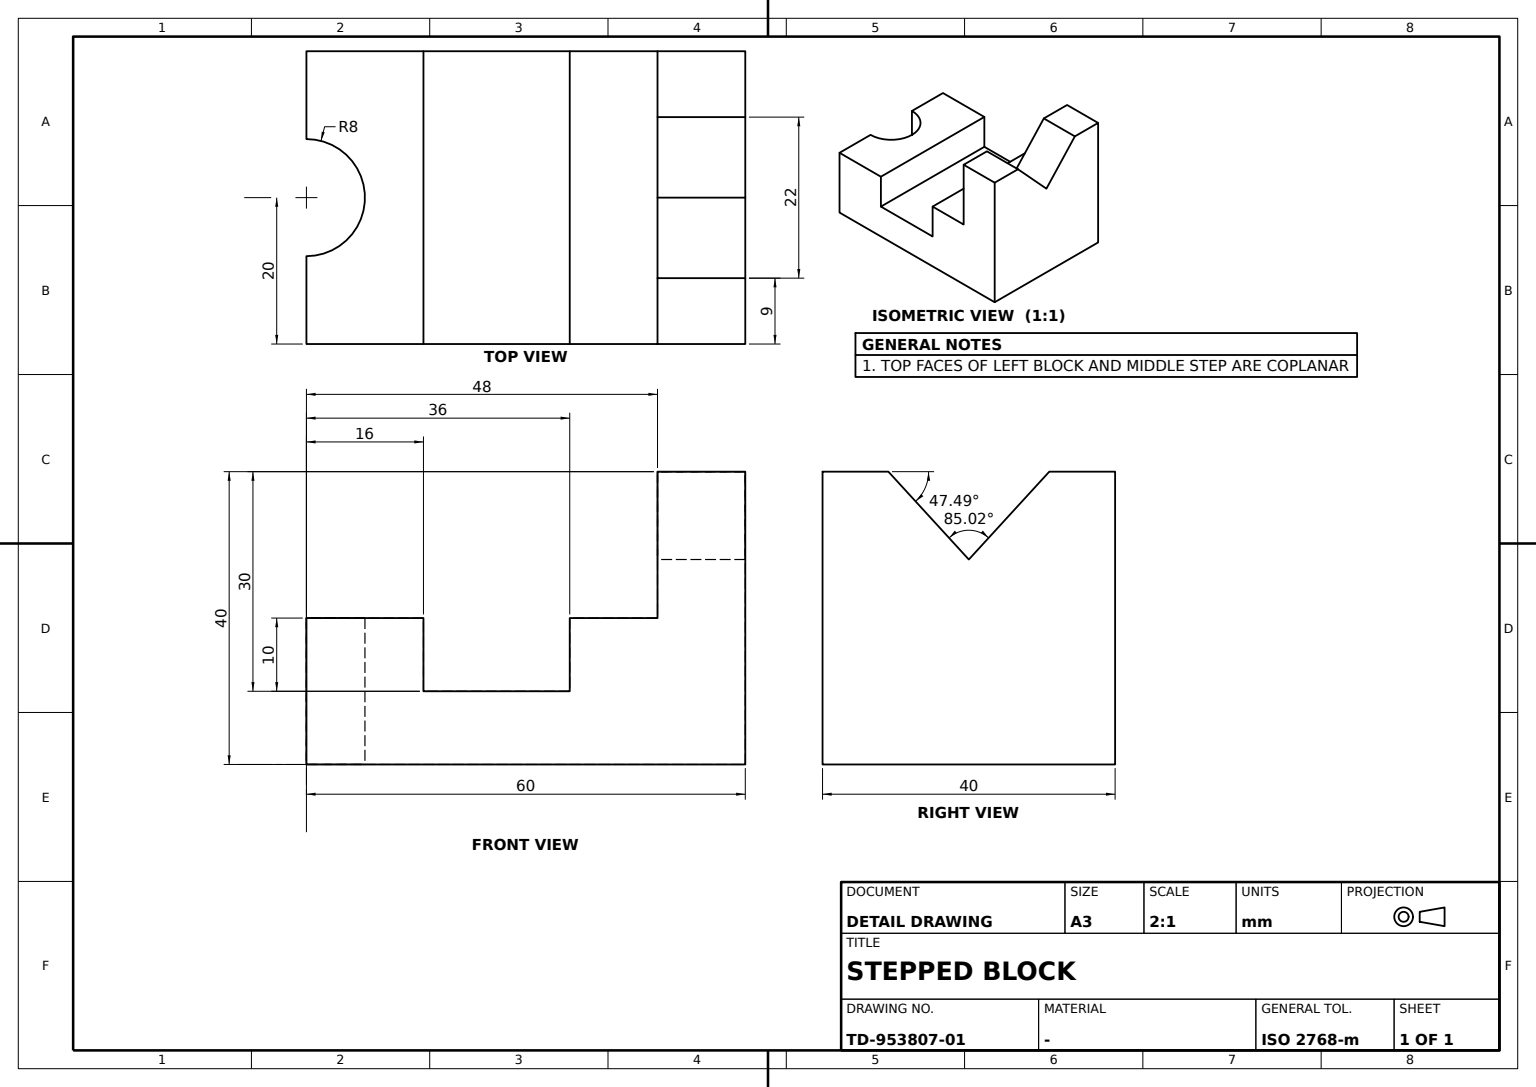
ISO-10303-21;
HEADER;
FILE_DESCRIPTION((''),'2;1');
FILE_NAME('','',(''),(''),'','','');
FILE_SCHEMA(('AUTOMOTIVE_DESIGN'));
ENDSEC;
DATA;
#1=APPLICATION_CONTEXT('');
#2=PRODUCT_CONTEXT('',#1,'mechanical');
#3=PRODUCT('','','',(#2));
#4=PRODUCT_DEFINITION_FORMATION('','',#3);
#5=PRODUCT_DEFINITION_CONTEXT('',#1,'design');
#6=PRODUCT_DEFINITION('','',#4,#5);
#7=PRODUCT_DEFINITION_SHAPE('','',#6);
#8=(LENGTH_UNIT()NAMED_UNIT(*)SI_UNIT(.MILLI.,.METRE.));
#9=(NAMED_UNIT(*)PLANE_ANGLE_UNIT()SI_UNIT($,.RADIAN.));
#10=(NAMED_UNIT(*)SI_UNIT($,.STERADIAN.)SOLID_ANGLE_UNIT());
#11=UNCERTAINTY_MEASURE_WITH_UNIT(LENGTH_MEASURE(0.005),#8,'distance_accuracy_value','');
#12=(GEOMETRIC_REPRESENTATION_CONTEXT(3)GLOBAL_UNCERTAINTY_ASSIGNED_CONTEXT((#11))GLOBAL_UNIT_ASSIGNED_CONTEXT((#8,#9,#10))REPRESENTATION_CONTEXT('',''));
#13=CARTESIAN_POINT('',(11.,30.,40.));
#14=VERTEX_POINT('',#13);
#15=CARTESIAN_POINT('',(11.,18.,40.));
#16=VERTEX_POINT('',#15);
#17=CARTESIAN_POINT('',(11.,37.,40.));
#18=DIRECTION('',(0.,-1.,0.));
#19=VECTOR('',#18,1000.);
#20=LINE('',#17,#19);
#21=EDGE_CURVE('',#14,#16,#20,.T.);
#22=ORIENTED_EDGE('',*,*,#21,.T.);
#23=CARTESIAN_POINT('',(20.,18.,40.));
#24=VERTEX_POINT('',#23);
#25=DIRECTION('',(-1.,0.,0.));
#26=VECTOR('',#25,1000.);
#27=LINE('',#23,#26);
#28=EDGE_CURVE('',#24,#16,#27,.T.);
#29=ORIENTED_EDGE('',*,*,#28,.F.);
#30=CARTESIAN_POINT('',(20.,30.,40.));
#31=VERTEX_POINT('',#30);
#32=DIRECTION('',(0.,1.,0.));
#33=VECTOR('',#32,1000.);
#34=LINE('',#23,#33);
#35=EDGE_CURVE('',#24,#31,#34,.T.);
#36=ORIENTED_EDGE('',*,*,#35,.T.);
#37=LINE('',#30,#26);
#38=EDGE_CURVE('',#31,#14,#37,.T.);
#39=ORIENTED_EDGE('',*,*,#38,.T.);
#40=EDGE_LOOP('',(#22,#29,#36,#39));
#41=FACE_BOUND('',#40,.T.);
#42=DIRECTION('',(0.,0.,1.));
#43=DIRECTION('',(1.,0.,0.));
#44=AXIS2_PLACEMENT_3D('',#23,#42,#43);
#45=PLANE('',#44);
#46=ADVANCED_FACE('',(#41),#45,.T.);
#47=CARTESIAN_POINT('',(-20.,18.,40.));
#48=VERTEX_POINT('',#47);
#49=CARTESIAN_POINT('',(-20.,30.,40.));
#50=VERTEX_POINT('',#49);
#51=LINE('',#47,#33);
#52=EDGE_CURVE('',#48,#50,#51,.T.);
#53=ORIENTED_EDGE('',*,*,#52,.F.);
#54=CARTESIAN_POINT('',(-11.,18.,40.));
#55=VERTEX_POINT('',#54);
#56=EDGE_CURVE('',#55,#48,#27,.T.);
#57=ORIENTED_EDGE('',*,*,#56,.F.);
#58=CARTESIAN_POINT('',(-11.,30.,40.));
#59=VERTEX_POINT('',#58);
#60=CARTESIAN_POINT('',(-11.,37.,40.));
#61=LINE('',#60,#19);
#62=EDGE_CURVE('',#59,#55,#61,.T.);
#63=ORIENTED_EDGE('',*,*,#62,.F.);
#64=EDGE_CURVE('',#59,#50,#37,.T.);
#65=ORIENTED_EDGE('',*,*,#64,.T.);
#66=EDGE_LOOP('',(#53,#57,#63,#65));
#67=FACE_BOUND('',#66,.T.);
#68=ADVANCED_FACE('',(#67),#45,.T.);
#69=CARTESIAN_POINT('',(-20.,18.,20.));
#70=VERTEX_POINT('',#69);
#71=CARTESIAN_POINT('',(-20.,18.,0.));
#72=VECTOR('',#42,1000.);
#73=LINE('',#71,#72);
#74=EDGE_CURVE('',#70,#48,#73,.T.);
#75=ORIENTED_EDGE('',*,*,#74,.T.);
#76=ORIENTED_EDGE('',*,*,#52,.T.);
#77=CARTESIAN_POINT('',(-20.,30.,0.));
#78=VERTEX_POINT('',#77);
#79=LINE('',#77,#72);
#80=EDGE_CURVE('',#78,#50,#79,.T.);
#81=ORIENTED_EDGE('',*,*,#80,.F.);
#82=CARTESIAN_POINT('',(-20.,-30.,0.));
#83=VERTEX_POINT('',#82);
#84=LINE('',#82,#33);
#85=EDGE_CURVE('',#83,#78,#84,.T.);
#86=ORIENTED_EDGE('',*,*,#85,.F.);
#87=CARTESIAN_POINT('',(-20.,-30.,20.));
#88=VERTEX_POINT('',#87);
#89=CARTESIAN_POINT('',(-20.,-30.,10.));
#90=DIRECTION('',(0.,0.,-1.));
#91=VECTOR('',#90,1000.);
#92=LINE('',#89,#91);
#93=EDGE_CURVE('',#88,#83,#92,.T.);
#94=ORIENTED_EDGE('',*,*,#93,.F.);
#95=CARTESIAN_POINT('',(-20.,-14.,20.));
#96=VERTEX_POINT('',#95);
#97=LINE('',#87,#33);
#98=EDGE_CURVE('',#88,#96,#97,.T.);
#99=ORIENTED_EDGE('',*,*,#98,.T.);
#100=CARTESIAN_POINT('',(-20.,-14.,10.));
#101=VERTEX_POINT('',#100);
#102=LINE('',#95,#91);
#103=EDGE_CURVE('',#96,#101,#102,.T.);
#104=ORIENTED_EDGE('',*,*,#103,.T.);
#105=CARTESIAN_POINT('',(-20.,6.,10.));
#106=VERTEX_POINT('',#105);
#107=CARTESIAN_POINT('',(-20.,30.,10.));
#108=LINE('',#107,#19);
#109=EDGE_CURVE('',#106,#101,#108,.T.);
#110=ORIENTED_EDGE('',*,*,#109,.F.);
#111=CARTESIAN_POINT('',(-20.,6.,20.));
#112=VERTEX_POINT('',#111);
#113=LINE('',#111,#91);
#114=EDGE_CURVE('',#112,#106,#113,.T.);
#115=ORIENTED_EDGE('',*,*,#114,.F.);
#116=CARTESIAN_POINT('',(-20.,30.,20.));
#117=LINE('',#116,#19);
#118=EDGE_CURVE('',#70,#112,#117,.T.);
#119=ORIENTED_EDGE('',*,*,#118,.F.);
#120=EDGE_LOOP('',(#75,#76,#81,#86,#94,#99,#104,#110,#115,#119));
#121=FACE_BOUND('',#120,.T.);
#122=CARTESIAN_POINT('',(-20.,0.,0.));
#123=AXIS2_PLACEMENT_3D('',#122,#43,#90);
#124=PLANE('',#123);
#125=ADVANCED_FACE('',(#121),#124,.F.);
#126=CARTESIAN_POINT('',(20.,18.,20.));
#127=VERTEX_POINT('',#126);
#128=CARTESIAN_POINT('',(20.,6.,20.));
#129=VERTEX_POINT('',#128);
#130=CARTESIAN_POINT('',(20.,30.,20.));
#131=LINE('',#130,#19);
#132=EDGE_CURVE('',#127,#129,#131,.T.);
#133=ORIENTED_EDGE('',*,*,#132,.F.);
#134=VECTOR('',#43,1000.);
#135=LINE('',#126,#134);
#136=EDGE_CURVE('',#70,#127,#135,.T.);
#137=ORIENTED_EDGE('',*,*,#136,.F.);
#138=ORIENTED_EDGE('',*,*,#118,.T.);
#139=LINE('',#128,#26);
#140=EDGE_CURVE('',#129,#112,#139,.T.);
#141=ORIENTED_EDGE('',*,*,#140,.F.);
#142=EDGE_LOOP('',(#133,#137,#138,#141));
#143=FACE_BOUND('',#142,.T.);
#144=AXIS2_PLACEMENT_3D('',#130,#90,#32);
#145=PLANE('',#144);
#146=ADVANCED_FACE('',(#143),#145,.F.);
#147=ORIENTED_EDGE('',*,*,#56,.T.);
#148=ORIENTED_EDGE('',*,*,#74,.F.);
#149=ORIENTED_EDGE('',*,*,#136,.T.);
#150=CARTESIAN_POINT('',(20.,18.,0.));
#151=LINE('',#150,#72);
#152=EDGE_CURVE('',#127,#24,#151,.T.);
#153=ORIENTED_EDGE('',*,*,#152,.T.);
#154=ORIENTED_EDGE('',*,*,#28,.T.);
#155=CARTESIAN_POINT('',(0.,18.,28.));
#156=VERTEX_POINT('',#155);
#157=CARTESIAN_POINT('',(-4.815094,18.,22.74717));
#158=DIRECTION('',(0.675724629,0.,0.73715414));
#159=VECTOR('',#158,1000.);
#160=LINE('',#157,#159);
#161=EDGE_CURVE('',#156,#16,#160,.T.);
#162=ORIENTED_EDGE('',*,*,#161,.F.);
#163=CARTESIAN_POINT('',(23.079245,18.,2.822642));
#164=DIRECTION('',(0.675724629,0.,-0.73715414));
#165=VECTOR('',#164,1000.);
#166=LINE('',#163,#165);
#167=EDGE_CURVE('',#55,#156,#166,.T.);
#168=ORIENTED_EDGE('',*,*,#167,.F.);
#169=EDGE_LOOP('',(#147,#148,#149,#153,#154,#162,#168));
#170=FACE_BOUND('',#169,.T.);
#171=AXIS2_PLACEMENT_3D('',#150,#18,#90);
#172=PLANE('',#171);
#173=ADVANCED_FACE('',(#170),#172,.T.);
#174=ORIENTED_EDGE('',*,*,#167,.T.);
#175=CARTESIAN_POINT('',(0.,30.,28.));
#176=VERTEX_POINT('',#175);
#177=CARTESIAN_POINT('',(0.,37.,28.));
#178=LINE('',#177,#19);
#179=EDGE_CURVE('',#156,#176,#178,.F.);
#180=ORIENTED_EDGE('',*,*,#179,.T.);
#181=CARTESIAN_POINT('',(23.079245,30.,2.822642));
#182=LINE('',#181,#165);
#183=EDGE_CURVE('',#59,#176,#182,.T.);
#184=ORIENTED_EDGE('',*,*,#183,.F.);
#185=ORIENTED_EDGE('',*,*,#62,.T.);
#186=EDGE_LOOP('',(#174,#180,#184,#185));
#187=FACE_BOUND('',#186,.T.);
#188=DIRECTION('',(-0.73715414,0.,-0.675724629));
#189=DIRECTION('',(-0.675724629,0.,0.73715414));
#190=AXIS2_PLACEMENT_3D('',#60,#188,#189);
#191=PLANE('',#190);
#192=ADVANCED_FACE('',(#187),#191,.F.);
#193=CARTESIAN_POINT('',(20.,-30.,0.));
#194=VERTEX_POINT('',#193);
#195=CARTESIAN_POINT('',(8.,-30.,0.));
#196=VERTEX_POINT('',#195);
#197=LINE('',#193,#26);
#198=EDGE_CURVE('',#194,#196,#197,.T.);
#199=ORIENTED_EDGE('',*,*,#198,.F.);
#200=CARTESIAN_POINT('',(20.,-30.,20.));
#201=VERTEX_POINT('',#200);
#202=CARTESIAN_POINT('',(20.,-30.,10.));
#203=LINE('',#202,#91);
#204=EDGE_CURVE('',#201,#194,#203,.T.);
#205=ORIENTED_EDGE('',*,*,#204,.F.);
#206=CARTESIAN_POINT('',(8.,-30.,20.));
#207=VERTEX_POINT('',#206);
#208=LINE('',#200,#26);
#209=EDGE_CURVE('',#201,#207,#208,.T.);
#210=ORIENTED_EDGE('',*,*,#209,.T.);
#211=CARTESIAN_POINT('',(8.,-30.,37.));
#212=LINE('',#211,#91);
#213=EDGE_CURVE('',#207,#196,#212,.T.);
#214=ORIENTED_EDGE('',*,*,#213,.T.);
#215=EDGE_LOOP('',(#199,#205,#210,#214));
#216=FACE_BOUND('',#215,.T.);
#217=AXIS2_PLACEMENT_3D('',#202,#32,#42);
#218=PLANE('',#217);
#219=ADVANCED_FACE('',(#216),#218,.F.);
#220=CARTESIAN_POINT('',(20.,-14.,20.));
#221=VERTEX_POINT('',#220);
#222=LINE('',#220,#26);
#223=EDGE_CURVE('',#221,#96,#222,.T.);
#224=ORIENTED_EDGE('',*,*,#223,.F.);
#225=CARTESIAN_POINT('',(20.,-14.,10.));
#226=VERTEX_POINT('',#225);
#227=LINE('',#220,#91);
#228=EDGE_CURVE('',#221,#226,#227,.T.);
#229=ORIENTED_EDGE('',*,*,#228,.T.);
#230=LINE('',#225,#134);
#231=EDGE_CURVE('',#101,#226,#230,.T.);
#232=ORIENTED_EDGE('',*,*,#231,.F.);
#233=ORIENTED_EDGE('',*,*,#103,.F.);
#234=EDGE_LOOP('',(#224,#229,#232,#233));
#235=FACE_BOUND('',#234,.T.);
#236=AXIS2_PLACEMENT_3D('',#220,#32,#42);
#237=PLANE('',#236);
#238=ADVANCED_FACE('',(#235),#237,.T.);
#239=ORIENTED_EDGE('',*,*,#114,.T.);
#240=CARTESIAN_POINT('',(20.,6.,10.));
#241=VERTEX_POINT('',#240);
#242=LINE('',#240,#26);
#243=EDGE_CURVE('',#241,#106,#242,.T.);
#244=ORIENTED_EDGE('',*,*,#243,.F.);
#245=LINE('',#128,#91);
#246=EDGE_CURVE('',#129,#241,#245,.T.);
#247=ORIENTED_EDGE('',*,*,#246,.F.);
#248=ORIENTED_EDGE('',*,*,#140,.T.);
#249=EDGE_LOOP('',(#239,#244,#247,#248));
#250=FACE_BOUND('',#249,.T.);
#251=AXIS2_PLACEMENT_3D('',#128,#32,#42);
#252=PLANE('',#251);
#253=ADVANCED_FACE('',(#250),#252,.F.);
#254=ORIENTED_EDGE('',*,*,#246,.T.);
#255=CARTESIAN_POINT('',(20.,30.,10.));
#256=LINE('',#255,#19);
#257=EDGE_CURVE('',#241,#226,#256,.T.);
#258=ORIENTED_EDGE('',*,*,#257,.T.);
#259=ORIENTED_EDGE('',*,*,#228,.F.);
#260=LINE('',#200,#33);
#261=EDGE_CURVE('',#201,#221,#260,.T.);
#262=ORIENTED_EDGE('',*,*,#261,.F.);
#263=ORIENTED_EDGE('',*,*,#204,.T.);
#264=CARTESIAN_POINT('',(20.,30.,0.));
#265=VERTEX_POINT('',#264);
#266=LINE('',#193,#33);
#267=EDGE_CURVE('',#194,#265,#266,.T.);
#268=ORIENTED_EDGE('',*,*,#267,.T.);
#269=LINE('',#264,#72);
#270=EDGE_CURVE('',#265,#31,#269,.T.);
#271=ORIENTED_EDGE('',*,*,#270,.T.);
#272=ORIENTED_EDGE('',*,*,#35,.F.);
#273=ORIENTED_EDGE('',*,*,#152,.F.);
#274=ORIENTED_EDGE('',*,*,#132,.T.);
#275=EDGE_LOOP('',(#254,#258,#259,#262,#263,#268,#271,#272,#273,#274));
#276=FACE_BOUND('',#275,.T.);
#277=CARTESIAN_POINT('',(20.,0.,0.));
#278=AXIS2_PLACEMENT_3D('',#277,#43,#90);
#279=PLANE('',#278);
#280=ADVANCED_FACE('',(#276),#279,.T.);
#281=ORIENTED_EDGE('',*,*,#223,.T.);
#282=ORIENTED_EDGE('',*,*,#98,.F.);
#283=CARTESIAN_POINT('',(-8.,-30.,20.));
#284=VERTEX_POINT('',#283);
#285=EDGE_CURVE('',#284,#88,#208,.T.);
#286=ORIENTED_EDGE('',*,*,#285,.F.);
#287=CARTESIAN_POINT('',(0.,-30.,20.));
#288=AXIS2_PLACEMENT_3D('',#287,#42,#43);
#289=CIRCLE('',#288,8.);
#290=EDGE_CURVE('',#207,#284,#289,.T.);
#291=ORIENTED_EDGE('',*,*,#290,.F.);
#292=ORIENTED_EDGE('',*,*,#209,.F.);
#293=ORIENTED_EDGE('',*,*,#261,.T.);
#294=EDGE_LOOP('',(#281,#282,#286,#291,#292,#293));
#295=FACE_BOUND('',#294,.T.);
#296=AXIS2_PLACEMENT_3D('',#200,#42,#43);
#297=PLANE('',#296);
#298=ADVANCED_FACE('',(#295),#297,.T.);
#299=ORIENTED_EDGE('',*,*,#213,.F.);
#300=ORIENTED_EDGE('',*,*,#290,.T.);
#301=CARTESIAN_POINT('',(-8.,-30.,0.));
#302=VERTEX_POINT('',#301);
#303=CARTESIAN_POINT('',(-8.,-30.,37.));
#304=LINE('',#303,#91);
#305=EDGE_CURVE('',#302,#284,#304,.F.);
#306=ORIENTED_EDGE('',*,*,#305,.F.);
#307=CARTESIAN_POINT('',(0.,-30.,0.));
#308=AXIS2_PLACEMENT_3D('',#307,#42,#43);
#309=CIRCLE('',#308,8.);
#310=EDGE_CURVE('',#196,#302,#309,.T.);
#311=ORIENTED_EDGE('',*,*,#310,.F.);
#312=EDGE_LOOP('',(#299,#300,#306,#311));
#313=FACE_BOUND('',#312,.T.);
#314=CARTESIAN_POINT('',(0.,-30.,37.));
#315=AXIS2_PLACEMENT_3D('',#314,#90,#25);
#316=CYLINDRICAL_SURFACE('',#315,8.);
#317=ADVANCED_FACE('',(#313),#316,.F.);
#318=ORIENTED_EDGE('',*,*,#305,.T.);
#319=ORIENTED_EDGE('',*,*,#285,.T.);
#320=ORIENTED_EDGE('',*,*,#93,.T.);
#321=EDGE_CURVE('',#302,#83,#197,.T.);
#322=ORIENTED_EDGE('',*,*,#321,.F.);
#323=EDGE_LOOP('',(#318,#319,#320,#322));
#324=FACE_BOUND('',#323,.T.);
#325=ADVANCED_FACE('',(#324),#218,.F.);
#326=ORIENTED_EDGE('',*,*,#85,.T.);
#327=LINE('',#264,#26);
#328=EDGE_CURVE('',#265,#78,#327,.T.);
#329=ORIENTED_EDGE('',*,*,#328,.F.);
#330=ORIENTED_EDGE('',*,*,#267,.F.);
#331=ORIENTED_EDGE('',*,*,#198,.T.);
#332=ORIENTED_EDGE('',*,*,#310,.T.);
#333=ORIENTED_EDGE('',*,*,#321,.T.);
#334=EDGE_LOOP('',(#326,#329,#330,#331,#332,#333));
#335=FACE_BOUND('',#334,.T.);
#336=AXIS2_PLACEMENT_3D('',#193,#42,#43);
#337=PLANE('',#336);
#338=ADVANCED_FACE('',(#335),#337,.F.);
#339=ORIENTED_EDGE('',*,*,#161,.T.);
#340=ORIENTED_EDGE('',*,*,#21,.F.);
#341=CARTESIAN_POINT('',(-4.815094,30.,22.74717));
#342=LINE('',#341,#159);
#343=EDGE_CURVE('',#176,#14,#342,.T.);
#344=ORIENTED_EDGE('',*,*,#343,.F.);
#345=ORIENTED_EDGE('',*,*,#179,.F.);
#346=EDGE_LOOP('',(#339,#340,#344,#345));
#347=FACE_BOUND('',#346,.T.);
#348=DIRECTION('',(0.73715414,0.,-0.675724629));
#349=DIRECTION('',(-0.675724629,0.,-0.73715414));
#350=AXIS2_PLACEMENT_3D('',#177,#348,#349);
#351=PLANE('',#350);
#352=ADVANCED_FACE('',(#347),#351,.F.);
#353=ORIENTED_EDGE('',*,*,#231,.T.);
#354=ORIENTED_EDGE('',*,*,#257,.F.);
#355=ORIENTED_EDGE('',*,*,#243,.T.);
#356=ORIENTED_EDGE('',*,*,#109,.T.);
#357=EDGE_LOOP('',(#353,#354,#355,#356));
#358=FACE_BOUND('',#357,.T.);
#359=AXIS2_PLACEMENT_3D('',#255,#90,#25);
#360=PLANE('',#359);
#361=ADVANCED_FACE('',(#358),#360,.F.);
#362=ORIENTED_EDGE('',*,*,#343,.T.);
#363=ORIENTED_EDGE('',*,*,#38,.F.);
#364=ORIENTED_EDGE('',*,*,#270,.F.);
#365=ORIENTED_EDGE('',*,*,#328,.T.);
#366=ORIENTED_EDGE('',*,*,#80,.T.);
#367=ORIENTED_EDGE('',*,*,#64,.F.);
#368=ORIENTED_EDGE('',*,*,#183,.T.);
#369=EDGE_LOOP('',(#362,#363,#364,#365,#366,#367,#368));
#370=FACE_BOUND('',#369,.T.);
#371=AXIS2_PLACEMENT_3D('',#264,#18,#90);
#372=PLANE('',#371);
#373=ADVANCED_FACE('',(#370),#372,.F.);
#374=CLOSED_SHELL('',(#46,#68,#125,#146,#173,#192,#219,#238,#253,#280,#298,#317,#325,#338,#352,#361,#373));
#375=MANIFOLD_SOLID_BREP('',#374);
#376=ADVANCED_BREP_SHAPE_REPRESENTATION('',(#375),#12);
#377=SHAPE_DEFINITION_REPRESENTATION(#7,#376);
ENDSEC;
END-ISO-10303-21;
